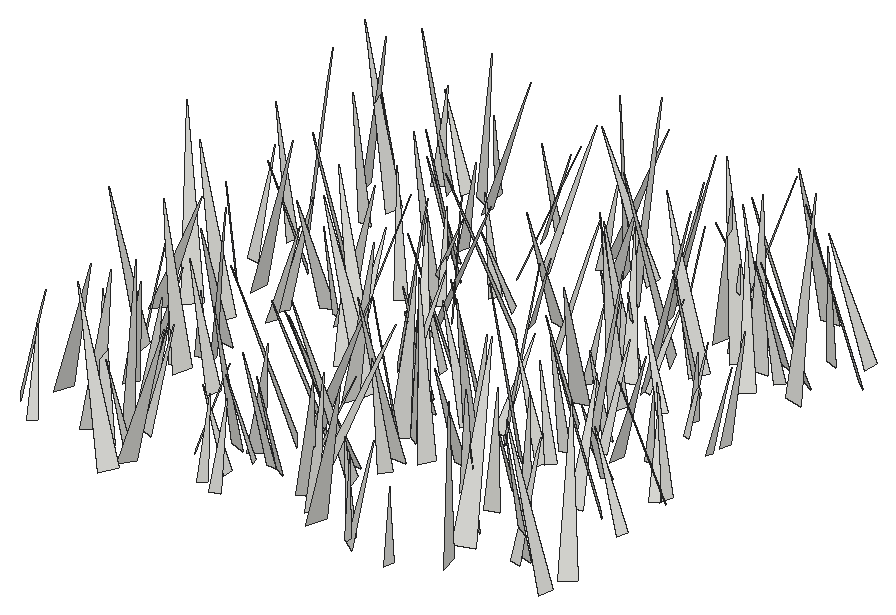
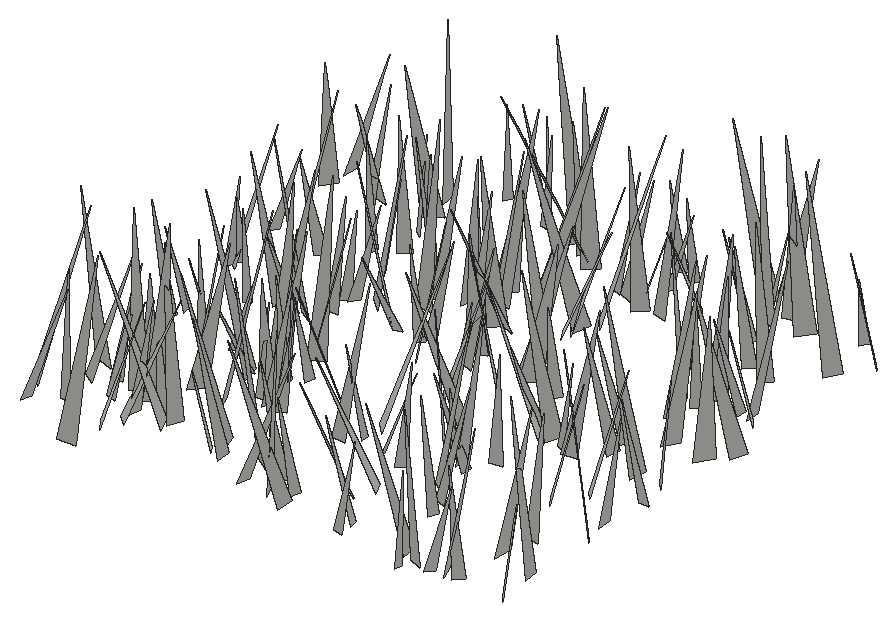
# SketchUp Ruby script. Lengths in inches.
U = 1.inch
M = Sketchup.active_model
def pt(a) = Geom::Point3d.new(a.map { |v| v * U })
def face(e, loops, mat)
  f = e.add_face(loops[0].map { |a| pt(a) })
  loops[1..].each { |l| e.add_face(l.map { |a| pt(a) }).erase! }
  f.material = f.back_material = mat if mat
  f
end
# faces: each face lists its corners as indices into pts; further lists are holes
def faces(e, pts, list, mat = nil) = list.each { |f| face(e, (f[0].is_a?(Array) ? f : [f]).map { |l| l.map { |i| pts[i] } }, mat) }
# xy, xz, yz: faces in a plane at the given z, y or x. An outline is a flat list of corners, or four numbers for a rectangle; further outlines are holes
def ring(l) = l.size == 4 ? [[l[0], l[1]], [l[2], l[1]], [l[2], l[3]], [l[0], l[3]]] : l.each_slice(2).to_a
def flat(e, list, mat, &to3) = list.each { |f| face(e, (f[0].is_a?(Array) ? f : [f]).map { |l| ring(l).map { |u, v| to3.(u, v) } }, mat) }
def xy(e, z, list, mat = nil) = flat(e, list, mat) { |x, y| [x, y, z] }
def xz(e, y, list, mat = nil) = flat(e, list, mat) { |x, z| [x, y, z] }
def yz(e, x, list, mat = nil) = flat(e, list, mat) { |y, z| [x, y, z] }
def lines(e, pts, list) = list.each { |a, b| e.add_line(pt(pts[a]), pt(pts[b])) }
# prism: a flat outline (further loops are holes) pulled along v
def prism(e, loops, v, mat = nil)
  f = face(e, loops, mat); d = Geom::Vector3d.new(v.map { |x| x * U })
  f.pushpull(f.normal.samedirection?(d) ? d.length : -d.length)
end
def box(e, o, s, mat = nil) = prism(e, [[o, [o[0] + s[0], o[1], o[2]], [o[0] + s[0], o[1] + s[1], o[2]], [o[0], o[1] + s[1], o[2]]]], [0, 0, s[2]], mat)
def at(x, y, z, deg = 0) = Geom::Transformation.translation(pt([x, y, z])) * Geom::Transformation.rotation(ORIGIN, Z_AXIS, deg.degrees)
def axes(o, x, y, z) = Geom::Transformation.new([*x, 0, *y, 0, *z, 0, *pt(o).to_a, 1])
def part(name) = M.definitions.add(name)
# library, detail: a bought-in or finely detailed component or shape, given as its bounding box
def library(name, o, s) = part(name).tap { |d| box(d.entities, o, s) }
def detail(e, o, s) = box(e.add_group.entities, o, s)
def put(e, d, t, mat = nil) = e.add_instance(d, t).tap { |i| i.material = mat if mat }
def group(e, t, mat = nil) = e.add_group.tap { |g| g.transformation = t; g.material = mat if mat }.entities
root = M.entities
c1 = part("fur_instance\#9")
p = [[0.8125,0,1.79],[0.67,-0.02,1.48],[0,-0.11,0],[0,0.11,0]]
faces(c1.entities,p,[[0,1,2,3]])
put(root,c1,axes([456.54,379.25,-21.66],[-6.24341,4.5177,1.05822],[4.50521,6.32678,-0.4296],[1.11019,-0.26807,7.69449]))
put(root,c1,axes([456.32,391.23,-21.66],[-5.31115,0.249,1.00047],[0.14264,5.37711,-0.58108],[1.02108,0.54405,5.28514]))
put(root,c1,axes([455.14,404.62,-21.66],[-2.6203,-2.567,1.06702],[-2.53846,2.80716,0.51965],[1.13325,0.35259,3.63117]))
put(root,c1,axes([455.45,360.47,-21.66],[3.51843,3.11531,1.14482],[3.25687,-3.56198,-0.31656],[-0.63919,-1.00114,4.68874]))
put(root,c1,axes([455.94,387.08,-21.66],[0.58745,4.61701,1.14714],[4.75417,-0.52722,-0.31264],[0.17496,-1.17604,4.64372]))
put(root,c1,axes([456.65,384.25,-21.66],[-2.76326,-3.0585,1.38467],[-3.15346,2.97986,0.28892],[1.15213,0.82059,4.11176]))
put(root,c1,axes([457.89,371.9,-21.66],[-6.59248,-1.12335,1.64682],[-1.04061,6.79216,0.46743],[1.70031,-0.1986,6.67115]))
put(root,c1,axes([455.68,400.69,-21.66],[6.8953,0.9557,1.85973],[1.13553,-7.09282,-0.56526],[-1.75571,-0.83402,6.93822]))
put(root,c1,axes([456.08,393.42,-21.66],[5.70767,4.90783,2.44546],[5.23724,-5.92496,-0.33273],[-1.62433,-1.85811,7.52021]))
put(root,c1,axes([454.9375,377.19,-21.66],[5.86888,-2.59714,0.14419],[-2.59865,-5.83866,0.60558],[0.11385,0.61201,6.38922]))
put(root,c1,axes([459.375,399.31,-21.66],[-7.31689,1.04904,1.18508],[0.99417,7.40794,-0.41938],[1.23147,0.25252,7.3798]))
put(root,c1,axes([457.24,372.65,-21.66],[3.19373,2.97376,0.94617],[2.91746,-3.32577,0.60507],[-1.10768,-0.18543,4.3217]))
put(root,c1,axes([458.28,358.33,-21.66],[-2.65941,2.49787,0.36396],[2.46932,2.68404,-0.37765],[0.52369,0.0288,3.62894]))
put(root,c1,axes([459.01,396.41,-21.66],[-0.51846,-5.08764,2.15235],[-5.51728,0.36879,-0.45728],[-0.27624,2.18298,5.0935]))
put(root,c1,axes([459.97,378.87,-21.66],[-6.35948,3.06032,1.72749],[3.24757,6.48259,0.47123],[1.34279,-1.18457,7.04176]))
put(root,c1,axes([459.87,388.57,-21.66],[-3.79874,-3.55526,0.6962],[-3.51199,3.8615,0.55657],[0.88909,0.06302,5.17306]))
put(root,c1,axes([460.84,404.07,-21.66],[-6.09908,-2.25868,1.59557],[-2.41433,6.23322,-0.4051],[1.3485,0.94419,6.49124]))
put(root,c1,axes([457.14,363.4,-21.66],[7.07591,-3.11018,0.05148],[-3.09924,-7.06002,-0.5432],[-0.26559,-0.47663,7.71016]))
put(root,c1,axes([458.8125,372.05,-21.66],[3.85375,-0.57416,0.66525],[-0.65849,-3.86826,0.47595],[-0.58191,0.57487,3.8671]))
put(root,c1,axes([459.56,404.24,-21.66],[2.82184,-3.33686,1.43593],[-3.57868,-2.86589,0.37288],[-0.62414,1.34588,4.35412]))
put(root,c1,axes([461.63,390.94,-21.66],[-4.56615,-2.82263,0.99228],[-2.92894,4.58662,-0.43101],[0.61084,0.89289,5.35081]))
put(root,c1,axes([458.95,384.02,-21.66],[7.358,-0.55238,1.16955],[-0.51092,-7.44716,-0.30295],[-1.18825,-0.21839,7.37248]))
put(root,c1,axes([461.96,404.66,-21.66],[-3.54918,2.04608,0.76374],[2.14815,3.53344,0.51649],[0.39398,-0.83357,4.06404]))
put(root,c1,axes([461.28,371.5,-21.66],[2.88206,-3.90926,2.29022],[-4.22914,-3.29495,-0.30223],[-1.62535,1.64154,4.8474]))
put(root,c1,axes([462.29,370.89,-21.66],[-6.37075,2.32719,2.17346],[2.54476,6.64308,0.34616],[1.91413,-1.08621,6.77365]))
put(root,c1,axes([460.4,367.22,-21.66],[4.90607,-3.46037,0.24315],[-3.44997,-4.91123,-0.28332],[-0.36191,-0.09172,5.99695]))
put(root,c1,axes([462.25,376.05,-21.66],[-0.34138,-6.1128,0.75859],[-6.1403,0.39794,0.44341],[0.48829,0.7305,6.10625]))
put(root,c1,axes([462.02,373.39,-21.66],[1.68223,-3.64936,0.16027],[-3.63941,-1.65928,0.41825],[0.31341,0.31999,3.9966]))
put(root,c1,axes([462.42,382.57,-21.66],[4.97792,-1.2009,1.19397],[-1.36113,-5.04298,0.6026],[-1.0075,0.87956,5.08515]))
put(root,c1,axes([462.67,366.3,-21.66],[2.7967,-3.72992,1.22325],[-3.91864,-2.74089,0.60164],[-0.23004,1.34365,4.62297]))
put(root,c1,axes([463.13,373.42,-21.66],[6.28919,2.00514,2.27548],[2.25266,-6.59596,-0.4138],[-2.03074,-1.10685,6.58812]))
put(root,c1,axes([462.73,380.8125,-21.66],[4.30722,-1.10997,0.82887],[-1.21703,-4.32511,0.53238],[-0.66174,0.72977,4.41597]))
put(root,c1,axes([463.48,404.46,-21.66],[-2.04646,-5.42862,2.85461],[-5.95901,2.47232,0.42963],[1.45222,2.49488,5.78561]))
put(root,c1,axes([462.46,359.96,-21.66],[5.72788,-5.11466,1.67521],[-5.30647,-5.77538,0.51083],[-0.89854,1.50329,7.66207]))
put(root,c1,axes([464.77,358.78,-21.66],[1.5886,-5.12639,3.23902],[-5.9044,-2.07062,-0.3813],[-1.38174,2.95423,5.35333]))
put(root,c1,axes([464.09,405.7,-21.66],[-3.40135,-0.48301,1.73948],[-0.24917,3.80046,0.56808],[1.78802,-0.38922,3.38818]))
put(root,c1,axes([464.74,384.86,-21.66],[1.62052,-5.44249,0.65001],[-5.43307,-1.68456,-0.55967],[-0.72449,0.45919,5.65098]))
put(root,c1,axes([466.17,369.7,-21.66],[-4.97411,1.9133,1.24146],[2.05101,5.05519,0.42681],[0.99764,-0.85328,5.31228]))
put(root,c1,axes([467.28,355.93,-21.66],[-6.20404,3.776,0.73856],[3.82283,6.20814,0.37243],[0.43544,-0.70326,7.25325]))
put(root,c1,axes([465.89,384.375,-21.66],[-1.30466,-3.28465,1.2487],[-3.51229,1.2605,-0.354],[0.10971,1.29326,3.5165]))
put(root,c1,axes([464.91,363.3,-21.66],[3.97041,-1.42005,1.05601],[-1.57618,-4.01704,0.5243],[-0.80459,0.86179,4.18399]))
put(root,c1,axes([466.41,359.32,-21.66],[-3.79793,-0.43925,1.06155],[-0.29859,3.91782,0.55288],[1.10936,-0.44932,3.78306]))
put(root,c1,axes([465.59,360.4,-21.66],[-2.07525,-6.86081,3.30693],[-7.48887,2.46229,0.40886],[1.38687,3.02978,7.15613]))
put(root,c1,axes([464.87,403.44,-21.66],[6.15775,0.09619,0.89999],[0.03195,-6.20791,0.44493],[-0.90455,0.43558,6.14241]))
put(root,c1,axes([466.04,362.05,-21.66],[1.29664,4.3065,0.97913],[4.41517,-1.23995,-0.39328],[0.1042,-1.05001,4.48024]))
put(root,c1,axes([467.77,396.24,-21.66],[-1.24841,-4.57565,0.91997],[-4.66472,1.19209,-0.401],[-0.15278,0.99186,4.72592]))
put(root,c1,axes([468.14,389.1875,-21.66],[-1.55203,4.86816,1.43833],[5.0761,1.479,0.47157],[-0.03172,-1.51332,5.08777]))
put(root,c1,axes([467.01,397.95,-21.66],[4.35751,-1.25814,0.68683],[-1.21703,-4.4086,-0.35441],[-0.75729,-0.15444,4.52164]))
put(root,c1,axes([467.15,383.69,-21.66],[6.16664,-2.56617,1.31423],[-2.70082,-6.22755,0.51287],[-1.00896,0.98602,6.65955]))
put(root,c1,axes([469.31,394.52,-21.66],[-3.91198,-5.41617,1.52932],[-5.50053,4.07361,0.35664],[1.19076,1.02376,6.67167]))
put(root,c1,axes([470.28,390.53,-21.66],[-6.61174,-0.50833,1.66504],[-0.62205,6.79727,-0.39495],[1.62598,0.53342,6.61948]))
put(root,c1,axes([469.25,382.67,-21.66],[-0.73079,4.32054,0.1844],[4.30671,0.74406,-0.36572],[0.39156,-0.12013,4.36662]))
put(root,c1,axes([467.59,357.74,-21.66],[6.355,-3.28716,0.66061],[-3.33311,-6.3472,0.48096],[-0.36352,0.73183,7.13864]))
put(root,c1,axes([470.93,378.75,-21.66],[-3.67286,3.55796,0.5072],[3.52102,3.70767,-0.51167],[0.72023,0.01818,5.08794]))
put(root,c1,axes([470.8,404.375,-21.66],[-0.62514,-3.66803,1.11265],[-3.82799,0.53943,-0.37244],[-0.19721,1.15663,3.70223]))
put(root,c1,axes([468.4,383.8,-21.66],[5.68273,3.19615,0.64935],[3.24559,-5.67036,-0.49352],[-0.32122,-0.74969,6.50117]))
put(root,c1,axes([471.07,390.32,-21.66],[-0.33834,3.74046,0.53618],[3.75079,0.26714,0.50319],[-0.45836,-0.57497,3.72187]))
put(root,c1,axes([469.18,391.38,-21.66],[3.86855,-0.79855,0.19754],[-0.81455,-3.85123,0.38332],[-0.11496,0.41562,3.93147]))
put(root,c1,axes([473.84,377.94,-21.66],[-6.13421,5.52562,0.24546],[5.52788,6.11218,0.5523],[-0.18784,-0.57446,8.23747]))
put(root,c1,axes([470.54,362.1,-21.66],[3.10796,2.24348,0.34109],[2.21254,-3.12436,0.38987],[-0.50422,0.11876,3.81322]))
put(root,c1,axes([470.72,402.69,-21.66],[4.18181,1.0835,0.53294],[1.13424,-4.18373,-0.39425],[-0.41412,-0.51766,4.30187]))
put(root,c1,axes([472.51,364.54,-21.66],[-2.15861,-6.19615,1.53511],[-6.31129,2.3146,0.46773],[0.95736,1.28794,6.5447]))
put(root,c1,axes([475.15,376.65,-21.66],[-7.32829,2.58062,0.59876],[2.60966,7.33524,0.32553],[0.45582,-0.50666,7.76257]))
put(root,c1,axes([473.3125,393.84,-21.66],[-3.08367,2.72536,1.78242],[3.08151,3.23588,0.38343],[1.05304,-1.48834,4.09751]))
put(root,c1,axes([474.41,361.08,-21.66],[-3.5972,0.42819,0.55364],[0.48536,3.61469,0.35791],[0.50428,-0.42464,3.60487]))
put(root,c1,axes([472.9,389.34,-21.66],[4.36466,2.86173,1.95624],[3.18404,-4.55325,-0.44325],[-1.3705,-1.46462,5.20032]))
put(root,c1,axes([475.32,368.01,-21.66],[-6.16047,-5.25921,0.96963],[-5.25018,6.22911,0.42963],[1.01736,0.29959,8.08864]))
put(root,c1,axes([474.88,363.6,-21.66],[-3.24657,-1.58505,0.39086],[-1.61743,3.24104,-0.29141],[0.22149,0.43432,3.60107]))
put(root,c1,axes([473.73,358.875,-21.66],[-2.42915,2.39744,1.43013],[2.49267,2.71628,-0.31959],[1.25681,-0.75355,3.39799]))
put(root,c1,axes([473.67,399.29,-21.66],[2.91229,5.1803,0.24137],[5.15397,-2.92189,0.52374],[-0.57474,0.04729,5.91968]))
put(root,c1,axes([472.66,397.36,-21.66],[5.42276,2.60915,0.23648],[2.58182,-5.41452,0.53583],[-0.44475,0.3811,5.9939]))
put(root,c1,axes([475.55,393.1875,-21.66],[-3.47043,-1.20582,0.35373],[-1.16309,3.47557,0.43669],[0.47575,-0.29913,3.64791]))
put(root,c1,axes([476.41,371.125,-21.66],[-4.47388,-2.50611,0.21033],[-2.51468,4.46372,-0.30343],[0.03476,0.36756,5.119]))
put(root,c1,axes([474.26,381.16,-21.66],[5.20843,4.28763,1.83578],[4.29945,-5.48037,0.60158],[-1.80791,-0.68076,6.71935]))
put(root,c1,axes([476.13,370.37,-21.66],[-4.87517,-3.87645,0.62854],[-3.83008,4.91477,0.6039],[0.86741,-0.08574,6.19915]))
put(root,c1,axes([476.33,363.81,-21.66],[-1.41742,-4.71426,1.18858],[-4.85717,1.31918,-0.56008],[-0.21176,1.29675,4.89077]))
put(root,c1,axes([473.3,386.41,-21.66],[6.47298,0.85818,0.33872],[0.84258,-6.4766,0.30739],[-0.37587,0.26066,6.52238]))
put(root,c1,axes([474.68,375.11,-21.66],[6.67765,-1.57713,2.05629],[-1.75682,-6.93326,0.38749],[-1.90506,0.86558,6.85042]))
put(root,c1,axes([474.16,364.71,-21.66],[4.15858,-4.6502,0.45845],[-4.67236,-4.14601,0.32855],[-0.05962,0.56087,6.22978]))
put(root,c1,axes([475.52,358.1875,-21.66],[-1.6026,3.32948,1.45838],[3.48573,1.8596,-0.41502],[1.03054,-1.11225,3.67172]))
put(root,c1,axes([477.46,383.69,-21.66],[-4.41159,-3.54695,0.73212],[-3.61607,4.3782,-0.57829],[0.20221,0.91078,5.63104]))
put(root,c1,axes([478.08,390.25,-21.66],[-5.65228,-5.31186,0.60473],[-5.29476,5.68375,0.43618],[0.73959,0.09466,7.74428]))
put(root,c1,axes([477.31,382.69,-21.66],[-3.67755,-0.2078,1.11626],[-0.0694,3.8179,0.48208],[1.13331,-0.4405,3.65173]))
put(root,c1,axes([477.3,363.58,-21.66],[-1.94034,-4.30134,0.80925],[-4.30819,2.03312,0.47669],[0.77193,0.53502,4.69459]))
put(root,c1,axes([476.8,401.9,-21.66],[3.29573,-2.04708,1.27302],[-2.29025,-3.33183,0.57152],[-0.75223,1.17531,3.83742]))
put(root,c1,axes([478.625,402.6,-21.66],[-6.27895,-2.5321,2.5957],[-2.9165,6.61067,-0.60625],[2.15482,1.56906,6.74309]))
put(root,c1,axes([479.55,377.18,-21.66],[-3.35316,6.39569,0.22234],[6.39729,3.34326,0.30873],[-0.17041,-0.34016,7.2148]))
put(root,c1,axes([478.91,379.2,-21.66],[-1.67954,-4.60165,1.09216],[-4.72861,1.65608,-0.29411],[0.09072,1.12742,4.88974]))
put(root,c1,axes([475.81,369.5,-21.66],[7.43524,-1.67911,0.29476],[-1.69435,-7.42416,0.44731],[-0.18841,0.50147,7.60934]))
put(root,c1,axes([476.43,403.58,-21.66],[6.73911,-0.51973,0.37006],[-0.5475,-6.72675,0.52311],[-0.32757,0.55072,6.73884]))
put(root,c1,axes([481.02,402.74,-21.66],[-6.42244,0.41118,0.57395],[0.45958,6.42194,0.54196],[0.53597,-0.57954,6.41273]))
put(root,c1,axes([478.06,392.21,-21.66],[3.62066,0.28745,0.41277],[0.34104,-3.60783,-0.479],[-0.36973,-0.51296,3.60033]))
put(root,c1,axes([479.46,393.49,-21.66],[-0.57876,-6.04691,0.53315],[-6.05695,0.61084,0.35302],[0.40347,0.49606,6.06428]))
put(root,c1,axes([478.1875,366.46,-21.66],[3.49532,2.40186,0.16337],[2.40303,-3.46356,-0.49202],[0.14512,-0.49771,4.21237]))
put(root,c1,axes([480.77,367.8,-21.66],[-1.44964,-7.72306,0.36058],[-7.72764,1.4358,-0.315],[-0.24346,0.41228,7.85162]))
put(root,c1,axes([478.83,400.83,-21.66],[3.52002,-2.83902,0.00242],[-2.82378,-3.50072,0.47096],[0.29379,0.3681,4.49764]))
put(root,c1,axes([482.51,365.6875,-21.66],[-7.47727,-2.4998,1.10622],[-2.44373,7.5564,0.55783],[1.22512,-0.18436,7.86431]))
put(root,c1,axes([480.15,372.875,-21.66],[2.22729,6.28936,0.04999],[6.2767,-2.22605,0.40869],[-0.40191,0.08939,6.65956]))
put(root,c1,axes([480.11,377.42,-21.66],[0.60186,-6.09784,0.10298],[-6.0697,-0.58883,0.60707],[0.59415,0.16161,6.09732]))
put(root,c1,axes([480.9,373.0625,-21.66],[4.75602,-4.66812,2.75377],[-5.20371,-4.95731,0.58378],[-1.51526,2.37234,6.63855]))
put(root,c1,axes([481.98,373.39,-21.66],[3.06348,4.37723,2.06786],[4.6001,-3.39453,0.37061],[-1.50841,-1.46222,5.32989]))
put(root,c1,axes([481.62,399.78,-21.66],[4.31651,6.80061,2.35568],[7.01576,-4.58865,0.3914],[-1.60519,-1.76799,8.04533]))
put(root,c1,axes([482.56,380.55,-21.66],[-4.52954,-3.25843,1.35312],[-3.24257,4.71245,0.49358],[1.39071,0.3748,5.55792]))
put(root,c1,axes([482.89,370.85,-21.66],[-4.49464,-4.79472,1.8462],[-5.03521,4.59856,-0.3156],[1.02201,1.56958,6.56442]))
put(root,c1,axes([483.625,377.61,-21.66],[-4.37438,2.14658,0.79892],[2.22863,4.38643,0.41683],[0.52851,-0.72986,4.85482]))
put(root,c1,axes([482.9,370.28,-21.66],[-0.40917,-7.70862,1.45343],[-7.84037,0.35495,-0.32469],[-0.25296,1.46762,7.71264]))
put(root,c1,axes([481.02,361.99,-21.66],[3.73638,-5.69312,0.32255],[-5.69521,-3.70663,0.54933],[0.28337,0.57053,6.78752]))
put(root,c1,axes([482.87,360.44,-21.66],[4.88657,-1.90502,2.44295],[-2.30886,-5.28158,0.49977],[-2.06549,1.39696,5.22091]))
put(root,c1,axes([483.39,368.3125,-21.66],[3.00214,-3.52749,1.91618],[-3.65397,-3.39209,-0.51969],[-1.66236,1.08552,4.60282]))
put(root,c1,axes([482.41,389.33,-21.66],[3.35621,4.76804,0.53975],[4.75729,-3.3924,0.38655],[-0.62744,-0.21695,5.81798]))
put(root,c1,axes([484.83,371.41,-21.66],[-6.58758,2.43197,1.48528],[2.355,6.75255,-0.6115],[1.60454,0.07391,6.99549]))
put(root,c1,axes([481.81,361.39,-21.66],[4.66085,6.54813,0.11631],[6.5407,-4.64683,-0.4912],[0.3329,-0.37945,8.02249]))
put(root,c1,axes([483.97,378.36,-21.66],[2.50338,-2.82714,1.30611],[-3.05988,-2.54469,0.35667],[-0.57944,1.22368,3.75931]))
put(root,c1,axes([485.69,392.09,-21.66],[-3.35833,-3.2337,1.73378],[-3.57177,3.41915,-0.54142],[0.83981,1.61055,4.63056]))
put(root,c1,axes([485.36,392.96,-21.66],[2.55514,-3.36467,0.69917],[-3.31318,-2.64324,-0.61213],[-0.91251,0.1757,4.18031]))
put(root,c1,axes([484.47,400.78,-21.66],[5.61379,-0.0924,1.25595],[-0.17391,-5.73971,0.3551],[-1.24727,0.38445,5.60331]))
put(root,c1,axes([486.77,392.54,-21.66],[-5.40914,1.11965,1.3835],[1.23539,5.5484,0.3398],[1.28121,-0.62292,5.51334]))
put(root,c1,axes([485.77,400.54,-21.66],[-2.4957,-1.61977,2.11338],[-2.18018,2.90599,-0.34732],[1.52869,1.50005,2.95492]))
put(root,c1,axes([484.07,359.42,-21.66],[7.12513,-3.29011,0.44393],[-3.26274,-7.13377,-0.50321],[-0.6135,-0.27186,7.83192]))
put(root,c1,axes([486.23,378.07,-21.66],[-0.08905,4.06249,0.07241],[4.03019,0.09752,-0.5148],[0.51634,-0.06053,4.03072]))
put(root,c1,axes([485.42,399.02,-21.66],[6.99973,1.86447,1.44835],[1.77883,-7.14461,0.6004],[-1.55233,0.22015,7.21886]))
put(root,c1,axes([487.35,359.375,-21.66],[0.08392,3.77547,1.67654],[4.10941,-0.2474,0.35143],[-0.42151,-1.66031,3.76001]))
put(root,c1,axes([486.81,374.34,-21.66],[-0.69172,-7.26259,1.83893],[-7.46362,0.82804,0.46276],[0.64909,1.78171,7.28077]))
put(root,c1,axes([486.66,387.88,-21.66],[3.38987,-1.12165,1.00676],[-1.27426,-3.45624,0.43994],[-0.80492,0.7478,3.54341]))
put(root,c1,axes([488.33,389.64,-21.66],[5.38161,2.47127,3.67462],[2.66712,-6.4254,0.41515],[-3.53503,-1.08568,5.90733]))
put(root,c1,axes([487.04,372.7,-21.66],[-0.08674,-5.50292,0.32115],[-5.49794,0.10952,0.39174],[0.3974,0.31411,5.48965]))
put(root,c1,axes([487.21,377.5625,-21.66],[5.30824,4.83924,1.79848],[4.88732,-5.54151,0.48577],[-1.6634,-0.83881,7.16657]))
put(root,c1,axes([489.05,389.91,-21.66],[-1.93628,5.55,0.46539],[5.55779,1.89356,0.54185],[-0.36056,-0.61659,5.85304]))
put(root,c1,axes([487.84,392.3125,-21.66],[-0.65259,-3.58567,0.77528],[-3.62638,0.74954,0.41412],[0.55447,0.682,3.62097]))
put(root,c1,axes([489.5,394.45,-21.66],[-7.3935,-3.44968,1.78048],[-3.41196,7.60131,0.55924],[1.85173,0.23234,8.13949]))
put(root,c1,axes([487.84,358.375,-21.66],[-1.12295,-3.74744,1.45837],[-3.89173,1.39395,0.58526],[1.01223,1.20198,3.86805]))
put(root,c1,axes([488.04,388.97,-21.66],[2.26375,-3.28304,0.92587],[-3.40814,-2.22313,0.4499],[-0.14199,1.01955,3.96238]))
put(root,c1,axes([489.95,376.04,-21.66],[4.02018,4.80904,4.066],[5.52928,-5.00439,0.45193],[-3.01434,-2.76593,6.25176]))
put(root,c1,axes([488.26,358.04,-21.66],[2.5994,3.80823,1.24151],[3.99906,-2.55122,-0.54734],[-0.2268,-1.33772,4.57819]))
put(root,c1,axes([488.11,385.28,-21.66],[2.21636,-6.61774,0.25451],[-6.61771,-2.20273,0.35418],[0.25535,0.35358,6.97003]))
put(root,c1,axes([490.18,382.41,-21.66],[-4.23671,-2.59002,0.97553],[-2.55905,4.34534,0.42292],[1.0541,0.13924,4.94763]))
put(root,c1,axes([489.75,369.91,-21.66],[4.11916,-1.93041,1.42636],[-1.9279,-4.34864,-0.31782],[-1.42975,0.30221,4.53795]))
put(root,c1,axes([491.55,376.51,-21.66],[-4.44101,1.77663,0.66677],[1.83519,4.45274,0.3588],[0.48276,-0.58331,4.76973]))
put(root,c1,axes([490.84,386.28,-21.66],[-6.55699,2.55506,2.62376],[2.8465,6.94107,0.35432],[2.30431,-1.30376,7.02829]))
put(root,c1,axes([492.32,393.98,-21.66],[-6.29408,3.56033,1.19684],[3.6784,6.31519,0.55815],[0.76008,-1.07993,7.20971]))
put(root,c1,axes([490.75,389.73,-21.66],[0.42201,3.83383,0.13948],[3.79822,-0.3978,-0.55775],[0.53966,-0.19825,3.81644]))
put(root,c1,axes([491.75,378.91,-21.66],[0.28904,-4.61969,1.68996],[-4.89331,-0.44312,-0.3744],[-0.50298,1.65624,4.61355]))
put(root,c1,axes([492.09,376.87,-21.66],[-2.34318,3.21724,1.23905],[3.43189,2.31946,0.46753],[0.3286,-1.2829,3.95253]))
put(root,c1,axes([490.32,399.07,-21.66],[6.63287,-1.89646,1.66739],[-1.83678,-6.83922,-0.47211],[-1.73291,-0.0097,6.88248]))
put(root,c1,axes([493.66,401.13,-21.66],[-3.87501,-4.05549,0.17386],[-4.05477,3.85598,-0.42797],[-0.18982,0.42113,5.59281]))
put(root,c1,axes([490.58,389.91,-21.66],[7.58691,1.58366,1.76713],[1.48707,-7.78642,0.59349],[-1.84915,0.23586,7.72768]))
put(root,c1,axes([493.68,399.74,-21.66],[-5.54027,1.19429,0.93196],[1.15956,5.61711,-0.30487],[0.97482,0.10593,5.65933]))
put(root,c1,axes([493.75,387.86,-21.66],[-2.71204,2.5664,0.21286],[2.56651,2.66825,0.52947],[-0.21147,-0.53003,3.69611]))
put(root,c1,axes([493.58,397.39,-21.66],[-6.05615,5.17907,2.30301],[5.46239,6.23254,0.34836],[1.51293,-1.77094,7.96105]))
put(root,c1,axes([492.17,357.77,-21.66],[3.31226,-1.52366,0.97308],[-1.49474,-3.45052,-0.31491],[-1.01694,0.10903,3.63228]))
put(root,c1,axes([492.66,371.85,-21.66],[-1.51621,-3.26203,0.55212],[-3.23761,1.58793,0.49084],[0.68086,0.28668,3.56354]))
put(root,c1,axes([492.16,398.23,-21.66],[2.05705,-3.40779,1.21765],[-3.60141,-2.06493,0.30505],[-0.3543,1.20424,3.9688]))
put(root,c1,axes([493.17,382.2,-21.66],[-0.82021,3.34867,1.94688],[3.86928,0.61559,0.57127],[-0.18046,-2.02092,3.4]))
put(root,c1,axes([494.51,402.65,-21.66],[-5.00716,-3.11226,0.75462],[-3.18598,4.98296,-0.58898],[0.32424,0.90067,5.86608]))
put(root,c1,axes([490.86,399.79,-21.66],[6.96857,2.87265,0.80723],[2.85827,-7.01507,0.2896],[-0.85676,-0.03815,7.53188]))
put(root,c1,axes([493.21,365.76,-21.66],[3.80415,1.70942,1.42934],[1.7089,-4.05302,0.29902],[-1.42996,-0.29602,4.15984]))
put(root,c1,axes([493.09,368.67,-21.66],[2.23095,-4.80055,1.901],[-5.14348,-2.24733,0.36107],[-0.45138,1.8816,5.28129]))
put(root,c1,axes([492.92,380.6,-21.66],[4.37398,5.97616,2.1686],[6.29129,-4.44766,-0.43255],[-0.91492,-2.01317,7.39318]))
put(root,c1,axes([493.97,380.51,-21.66],[0.66695,4.37993,0.08385],[4.36286,-0.67176,0.3871],[-0.39533,-0.02429,4.41347]))
put(root,c1,axes([494.55,391.22,-21.66],[4.53456,1.85789,3.16607],[2.55783,-5.20835,-0.60709],[-2.63311,-1.85992,4.86266]))
put(root,c1,axes([494.11,365.87,-21.66],[-2.25784,-3.06403,1.232],[-3.11024,2.47464,0.4545],[1.1102,0.70132,3.77883]))
put(root,c1,axes([494.85,363.24,-21.66],[-3.53884,7.24303,1.02774],[7.25201,3.62348,-0.56563],[0.96238,-0.67082,8.04145]))
put(root,c1,axes([494.83,406.25,-21.66],[0.47812,-7.3143,1.47747],[-7.45136,-0.54714,-0.29732],[-0.39895,1.45332,7.32388]))
put(root,c1,axes([495.06,370.09,-21.66],[4.42317,-1.03576,2.17466],[-1.28949,-4.85884,0.30856],[-2.03449,0.82776,4.53233]))
put(root,c1,axes([496.67,394.2,-21.66],[-4.29612,3.71614,0.38084],[3.69784,4.31285,-0.36964],[0.52979,0.03157,5.66831]))
put(root,c1,axes([495.29,397.09,-21.66],[1.282,-6.99581,3.06835],[-7.6361,-1.26107,0.31524],[-0.21483,3.07701,7.10532]))
put(root,c1,axes([495.56,360.56,-21.66],[-6.42267,-1.42598,3.31634],[-1.29179,7.22813,0.60623],[3.37087,0.05298,6.55107]))
put(root,c1,axes([496.43,398.97,-21.66],[-1.84979,-4.95748,0.73449],[-4.97918,1.90688,0.3307],[0.56907,0.57009,5.281]))
put(root,c1,axes([496.625,377.78,-21.66],[1.2889,-4.23263,0.01136],[-4.22076,-1.28617,-0.32791],[-0.31699,-0.08469,4.41236]))
put(root,c1,axes([496.32,388.37,-21.66],[3.38817,-1.89067,0.4047],[-1.85762,-3.4096,-0.37677],[-0.53632,-0.13453,3.86165]))
put(root,c1,axes([497.3,386.2,-21.66],[1.47589,3.3854,0.35503],[3.34161,-1.51469,0.55196],[-0.64858,-0.1002,3.65165]))
put(root,c1,axes([497.7,396.73,-21.66],[1.52237,-3.55739,1.37163],[-3.65271,-1.78416,-0.57315],[-1.09275,1.00785,3.82677]))
put(root,c1,axes([497.6,372.82,-21.66],[-1.60174,4.9541,0.61833],[4.97114,1.64265,-0.28364],[0.46172,-0.4996,5.19887]))
put(root,c1,axes([495.43,380.45,-21.66],[5.75538,-1.33671,0.29214],[-1.31847,-5.75568,-0.36093],[-0.36579,-0.28603,5.89753]))
put(root,c1,axes([497.57,381.57,-21.66],[0.85171,-3.4207,0.8533],[-3.50883,-0.73716,0.54719],[0.34265,0.95401,3.48241]))
put(root,c1,axes([499.51,397.74,-21.66],[-3.13069,-4.74867,0.6646],[-4.79451,3.11096,-0.35688],[0.06511,0.75154,5.67659]))
put(root,c1,axes([499.54,373.46,-21.66],[-4.76298,-4.61729,1.21885],[-4.61962,4.89113,0.47635],[1.20999,0.49843,6.61653]))
put(root,c1,axes([499.65,364.59,-21.66],[-2.15143,-4.58063,1.63472],[-4.86135,2.07952,-0.57094],[0.14745,1.72526,5.02841]))
put(root,c1,axes([498.79,401.43,-21.66],[-1.48378,-4.80354,1.85374],[-5.06695,1.70492,0.36217],[0.91449,1.65264,5.01442]))
put(root,c1,axes([499.24,363.75,-21.66],[1.25627,4.75609,0.70963],[4.78282,-1.31187,0.32531],[-0.49861,-0.60066,4.90844]))
put(root,c1,axes([501.26,402.91,-21.66],[-5.40823,0.65228,0.52882],[0.69912,5.40686,0.48075],[0.46513,-0.5426,5.42617]))
put(root,c1,axes([500.125,395.27,-21.66],[2.12447,7.8086,2.15105],[8.03257,-2.31646,0.47574],[-1.03873,-1.94278,8.07844]))
put(root,c1,axes([502.44,400.33,-21.66],[-5.20648,-5.71637,1.32602],[-5.85189,5.18966,-0.6046],[0.43665,1.3904,7.70836]))
put(root,c1,axes([501.52,377.22,-21.66],[-2.57238,2.98987,0.10946],[2.97729,2.57237,-0.29516],[0.29502,0.10983,3.93311]))
put(root,c1,axes([500.25,385.28,-21.66],[3.57631,0.31891,0.97988],[0.16002,-3.66803,0.60973],[-1.01797,0.54376,3.53835]))
put(root,c1,axes([501.83,377.97,-21.66],[-3.65311,-4.50937,0.62916],[-4.48426,3.70309,0.50402],[0.78847,0.16789,5.78149]))
put(root,c1,axes([500.41,386.98,-21.66],[4.80103,-0.44543,1.50068],[-0.59366,-4.99749,0.41591],[-1.44845,0.57184,4.80368]))
put(root,c1,axes([502.05,378.1,-21.66],[-4.36363,0.98227,0.81119],[0.91976,4.432,-0.41906],[0.88144,0.23814,4.45315]))
put(root,c1,axes([502.77,371.92,-21.66],[-3.82314,1.91513,0.41484],[1.95484,3.79049,0.51675],[0.13566,-0.64863,4.24466]))
put(root,c1,axes([503.81,361.65,-21.66],[-6.67851,0.63047,0.27765],[0.60623,6.66388,-0.54986],[0.32721,0.52189,6.68563]))
put(root,c1,axes([503.88,364.09,-21.66],[-5.08982,4.44528,0.70369],[4.40622,5.13821,-0.58816],[0.91699,-0.01575,6.73207]))
